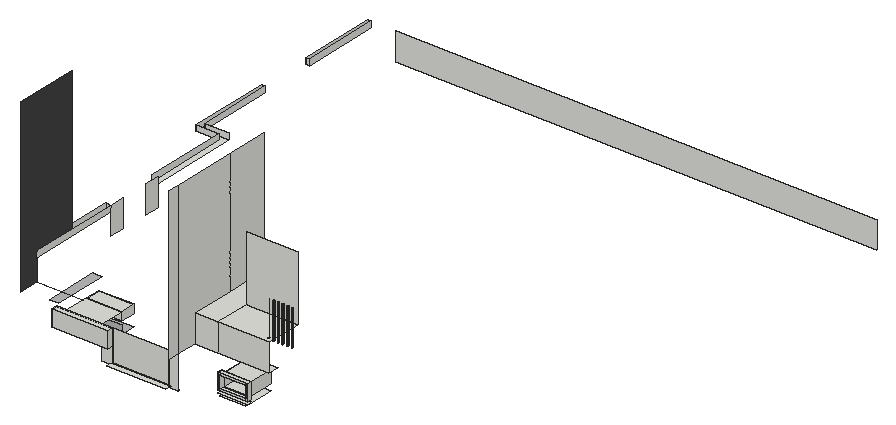
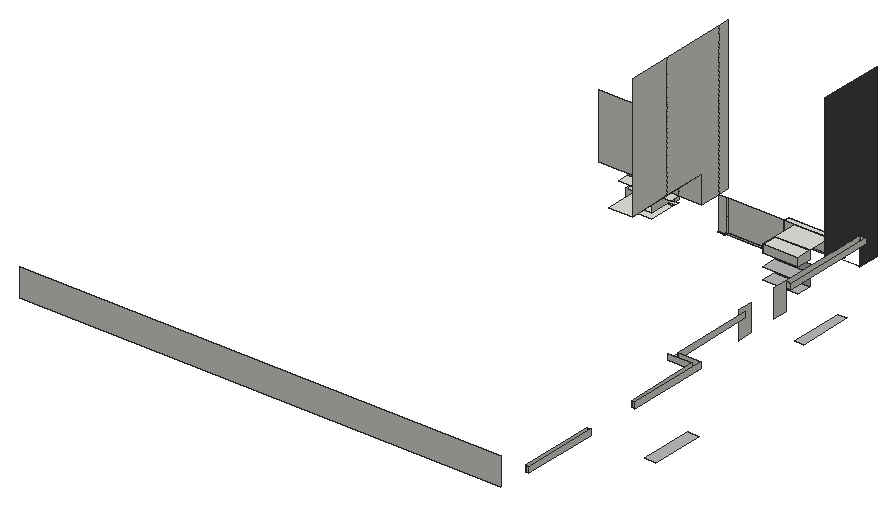
# SketchUp Ruby script. Lengths in inches.
U = 1.inch
M = Sketchup.active_model
def pt(a) = Geom::Point3d.new(a.map { |v| v * U })
def face(e, loops, mat)
  f = e.add_face(loops[0].map { |a| pt(a) })
  loops[1..].each { |l| e.add_face(l.map { |a| pt(a) }).erase! }
  f.material = f.back_material = mat if mat
  f
end
# faces: each face lists its corners as indices into pts; further lists are holes
def faces(e, pts, list, mat = nil) = list.each { |f| face(e, (f[0].is_a?(Array) ? f : [f]).map { |l| l.map { |i| pts[i] } }, mat) }
# xy, xz, yz: faces in a plane at the given z, y or x. An outline is a flat list of corners, or four numbers for a rectangle; further outlines are holes
def ring(l) = l.size == 4 ? [[l[0], l[1]], [l[2], l[1]], [l[2], l[3]], [l[0], l[3]]] : l.each_slice(2).to_a
def flat(e, list, mat, &to3) = list.each { |f| face(e, (f[0].is_a?(Array) ? f : [f]).map { |l| ring(l).map { |u, v| to3.(u, v) } }, mat) }
def xy(e, z, list, mat = nil) = flat(e, list, mat) { |x, y| [x, y, z] }
def xz(e, y, list, mat = nil) = flat(e, list, mat) { |x, z| [x, y, z] }
def yz(e, x, list, mat = nil) = flat(e, list, mat) { |y, z| [x, y, z] }
def lines(e, pts, list) = list.each { |a, b| e.add_line(pt(pts[a]), pt(pts[b])) }
# prism: a flat outline (further loops are holes) pulled along v
def prism(e, loops, v, mat = nil)
  f = face(e, loops, mat); d = Geom::Vector3d.new(v.map { |x| x * U })
  f.pushpull(f.normal.samedirection?(d) ? d.length : -d.length)
end
def box(e, o, s, mat = nil) = prism(e, [[o, [o[0] + s[0], o[1], o[2]], [o[0] + s[0], o[1] + s[1], o[2]], [o[0], o[1] + s[1], o[2]]]], [0, 0, s[2]], mat)
def at(x, y, z, deg = 0) = Geom::Transformation.translation(pt([x, y, z])) * Geom::Transformation.rotation(ORIGIN, Z_AXIS, deg.degrees)
def axes(o, x, y, z) = Geom::Transformation.new([*x, 0, *y, 0, *z, 0, *pt(o).to_a, 1])
def part(name) = M.definitions.add(name)
# library, detail: a bought-in or finely detailed component or shape, given as its bounding box
def library(name, o, s) = part(name).tap { |d| box(d.entities, o, s) }
def detail(e, o, s) = box(e.add_group.entities, o, s)
def put(e, d, t, mat = nil) = e.add_instance(d, t).tap { |i| i.material = mat if mat }
def group(e, t, mat = nil) = e.add_group.tap { |g| g.transformation = t; g.material = mat if mat }.entities
root = M.entities
M.materials.add("Generic\#2").color = [186, 186, 186]
M.materials.add("[Granite Dark Gray]").color = [68, 67, 67]
c1 = part("Group\#1")
xy(c1.entities,0,[[0,0,46.77,20.375]])
xz(c1.entities,0,[[0,0,46.77,11.0625]])
xy(root,943.1875,[[157.47,97.25,170.35,98],[249.19,97.25,259.3125,98]])
xy(root,943.6875,[[157.47,97.25,170.35,98],[249.19,97.25,259.3125,98]])
xy(root,945.84,[[170.35,89.25,249.19,97.25],[171.66,97.25,172.16,98],[247.01,97.25,247.51,98]])
xy(root,946,[[0,454.08,15.3125,525.8]],"Generic\#2")
xy(root,946.25,[[36.4375,161.95,48.5,234.18]],"Generic\#2")
xy(root,957.08,[[314.83,97.5,349.58,103.5],[314.83,103.5,349.58,138.74]])
xy(root,959.57,[[312.34,97.5,352.07,103.5]])
xy(root,962.59,[[312.34,97.5,352.07,103.5]])
xy(root,965.08,[[314.83,97.5,349.58,103.5],[314.83,103.5,349.58,138.74]])
xy(root,966.17,[[96.98,89.5625,171.66,97.25]])
xy(root,981.95,[[314.83,97.5,349.58,103.5],[314.83,103.5,349.58,138.74]])
xy(root,984.44,[[312.34,97.5,352.07,103.5]])
xy(root,987.75,[[96.98,89.5625,171.66,97.25],[110.7,97.25,157.47,130.3125],[171.66,97.25,172.16,98],[247.01,97.25,247.51,98],[290.4375,124.5,359.25,138.74],
  [110.7,130.3125,157.47,150.6875]])
xy(root,1016.8125,[[41,124.5,48.5,249],[41,326.1875,41,438.6875,10.5,438.6875,10.5,547.73,15.3125,547.73,15.3125,446.1875,48.5,446.1875,48.5,326.1875],[10.5,621.86,15.3125,724.5]])
xy(root,1024.6875,[[259.3125,124.5,290.4375,241.25],[[290.4375,124.5,359.25,172.5],[353.98,129.75,353.77,129.78,353.57,129.86,353.41,129.99,353.28,130.16,353.2,130.36,353.17,130.57,353.2,130.78,353.28,130.97,353.41,131.14,353.57,131.27,353.77,131.35,353.98,131.38,354.19,131.35,354.39,131.27,354.56,131.14,354.68,130.97,354.77,130.78,354.79,130.57,354.77,130.36,354.68,130.16,354.56,129.99,354.39,129.86,354.19,129.78]],[353.98,129.75,354.19,129.78,354.39,129.86,354.56,129.99,354.68,130.16,354.77,130.36,354.79,130.57,354.77,130.78,354.68,130.97,354.56,131.14,354.39,131.27,354.19,131.35,353.98,131.38,353.77,131.35,353.57,131.27,353.41,131.14,353.28,130.97,353.2,130.78,353.17,130.57,353.2,130.36,353.28,130.16,353.41,129.99,353.57,129.86,353.77,129.78],[360.79,129.75,360.58,129.78,360.39,129.86,360.22,129.99,360.09,130.16,360.01,130.36,359.98,130.57,360.01,130.78,360.09,130.97,360.22,131.14,360.39,131.27,360.58,131.35,360.79,131.38,361,131.35,361.2,131.27,361.37,131.14,361.5,130.97,361.58,130.78,361.61,130.57,361.58,130.36,361.5,130.16,361.37,129.99,361.2,129.86,361,129.78],[366.79,129.75,366.58,129.78,366.39,129.86,366.22,129.99,366.09,130.16,366.01,130.36,365.98,130.57,366.01,130.78,366.09,130.97,366.22,131.14,366.39,131.27,366.58,131.35,366.79,131.38,367,131.35,367.2,131.27,367.37,131.14,367.5,130.97,367.58,130.78,367.61,130.57,367.58,130.36,367.5,130.16,367.37,129.99,367.2,129.86,367,129.78],
  [372.73,129.75,372.52,129.78,372.32,129.86,372.16,129.99,372.03,130.16,371.95,130.36,371.92,130.57,371.95,130.78,372.03,130.97,372.16,131.14,372.32,131.27,372.52,131.35,372.73,131.38,372.94,131.35,373.14,131.27,373.31,131.14,373.43,130.97,373.52,130.78,373.54,130.57,373.52,130.36,373.43,130.16,373.31,129.99,373.14,129.86,372.94,129.78],[378.98,129.75,378.77,129.78,378.57,129.86,378.41,129.99,378.28,130.16,378.2,130.36,378.17,130.57,378.2,130.78,378.28,130.97,378.41,131.14,378.57,131.27,378.77,131.35,378.98,131.38,379.19,131.35,379.39,131.27,379.56,131.14,379.68,130.97,379.77,130.78,379.79,130.57,379.77,130.36,379.68,130.16,379.56,129.99,379.39,129.86,379.19,129.78],[385.23,129.75,385.02,129.78,384.82,129.86,384.66,129.99,384.53,130.16,384.45,130.36,384.42,130.57,384.45,130.78,384.53,130.97,384.66,131.14,384.82,131.27,385.02,131.35,385.23,131.38,385.44,131.35,385.64,131.27,385.81,131.14,385.93,130.97,386.02,130.78,386.04,130.57,386.02,130.36,385.93,130.16,385.81,129.99,385.64,129.86,385.44,129.78]])
xz(root,89.5625,[[96.98,966.17,171.66,987.75]])
xz(root,97.25,[[157.47,943.6875,170.35,943.6875,170.35,945.84,171.66,945.84,171.66,966.17,157.47,966.17],[170.35,943.6875,171.66,945.84],[171.66,943.6875,247.01,945.84],[247.01,943.6875,249.19,945.84],[249.19,943.6875,259.3125,943.6875,259.3125,987.75,247.51,987.75,247.51,945.84,249.19,945.84],
  [172.16,945.84,247.01,987.75],[96.98,966.17,110.7,987.75],[110.7,966.17,157.47,987.75],[157.47,966.17,171.66,987.75]])
xz(root,97.5,[[[312.34,962.59,352.07,984.44],[314.83,965.08,349.58,981.95]]])
xz(root,98,[[157.47,943.1875,170.35,943.6875],[249.19,943.1875,259.3125,943.6875],[171.66,945.84,172.16,987.75],[247.01,945.84,247.51,987.75]])
xz(root,103.5,[[[312.34,962.59,352.07,984.44],[314.83,965.08,349.58,981.95]]])
xz(root,124.5,[[259.3125,987.75,290.4375,1024.6875],[290.4375,987.75,359.25,1024.6875],[41,1016.8125,48.5,1024.6875]])
xz(root,150.6875,[[110.7,976.6875,157.47,987.75]])
xz(root,172.5,[[290.4375,1024.6875,359.25,1111.375]])
xz(root,249,[[41,1016.8125,48.5,1024.6875]])
xz(root,438.6875,[[10.5,1016.8125,41,1024.6875]])
xz(root,446.1875,[[15.3125,1016.8125,48.5,1024.6875]])
xz(root,547.73,[[10.5,1016.8125,15.3125,1024.6875]])
xz(root,621.86,[[10.5,1016.8125,15.3125,1024.6875]])
xz(root,724.5,[[48.5,987.75,690.4375,1024.6875],[10.5,1016.8125,15.3125,1024.6875]])
yz(root,10.5,[[438.6875,1016.8125,547.73,1024.6875],[621.86,1016.8125,724.5,1024.6875]])
yz(root,15.3125,[[446.1875,1016.8125,547.73,1024.6875],[621.86,1016.8125,724.5,1024.6875]])
yz(root,41,[[124.5,1016.8125,249,1024.6875],[326.1875,1016.8125,438.6875,1024.6875]])
yz(root,48.5,[[249,987.75,268.32,1024.6875],[306.87,987.75,326.1875,1024.6875],[124.5,1016.8125,249,1024.6875]])
yz(root,48.5,[[97.25,987.75,97.25,1214.9375,183.25,1214.9375,183.25,1024.6875,124.5,1024.6875,124.5,987.75]],"[Granite Dark Gray]")
yz(root,96.98,[[89.5625,966.17,97.25,987.75]])
yz(root,110.7,[[130.3125,976.6875,150.6875,987.75]])
yz(root,157.47,[[130.3125,976.6875,150.6875,987.75]])
yz(root,170.35,[[97.25,943.1875,98,943.6875]])
yz(root,171.66,[[97.25,945.84,98,966.17],[89.5625,966.17,97.25,987.75],[97.25,966.17,98,987.75]])
yz(root,172.16,[[97.25,945.84,98,966.17],[97.25,966.17,98,987.75]])
yz(root,247.01,[[97.25,945.84,98,966.17],[97.25,966.17,98,987.75]])
yz(root,247.51,[[97.25,945.84,98,966.17],[97.25,966.17,98,987.75]])
yz(root,249.19,[[97.25,943.1875,98,943.6875]])
yz(root,259.3125,[[81.125,987.75,97.25,1189.3125],[97.25,987.75,97.25,1189.3125,183.25,1189.3125,183.25,1024.6875,124.5,1024.6875,124.5,987.75],[183.25,1024.6875,241.25,1189.3125]])
yz(root,312.34,[[97.5,962.59,103.5,984.44]])
yz(root,314.83,[[97.5,965.08,103.5,981.95],[103.5,965.08,138.74,981.95]])
yz(root,349.58,[[97.5,965.08,103.5,981.95],[103.5,965.08,138.74,981.95]])
yz(root,352.07,[[97.5,962.59,103.5,984.44]])
p = [[360.39,129.86,1024.6875],[360.58,129.78,1024.6875],[360.58,129.78,1072.38],[360.39,129.86,1072.38],[360.79,129.75,1024.6875],[360.79,129.75,1072.38],
  [361,129.78,1024.6875],[361,129.78,1072.38],[361.2,129.86,1024.6875],[361.2,129.86,1072.38],[366.39,129.86,1024.6875],[366.58,129.78,1024.6875],
  [366.58,129.78,1072.38],[366.39,129.86,1072.38],[366.79,129.75,1024.6875],[366.79,129.75,1072.38],[367,129.78,1024.6875],[367,129.78,1072.38],
  [367.2,129.86,1024.6875],[367.2,129.86,1072.38],[372.32,129.86,1024.6875],[372.52,129.78,1024.6875],[372.52,129.78,1072.38],[372.32,129.86,1072.38],
  [372.73,129.75,1024.6875],[372.73,129.75,1072.38],[372.94,129.78,1024.6875],[372.94,129.78,1072.38],[373.14,129.86,1024.6875],[373.14,129.86,1072.38],
  [378.57,129.86,1024.6875],[378.77,129.78,1024.6875],[378.77,129.78,1072.38],[378.57,129.86,1072.38],[378.98,129.75,1024.6875],[378.98,129.75,1072.38],
  [379.19,129.78,1024.6875],[379.19,129.78,1072.38],[379.39,129.86,1024.6875],[379.39,129.86,1072.38],[384.82,129.86,1024.6875],[385.02,129.78,1024.6875],
  [385.02,129.78,1072.38],[384.82,129.86,1072.38],[385.23,129.75,1024.6875],[385.23,129.75,1072.38],[385.44,129.78,1024.6875],[385.44,129.78,1072.38],
  [385.64,129.86,1024.6875],[385.64,129.86,1072.38],[360.22,129.99,1024.6875],[360.22,129.99,1072.38],[361.37,129.99,1024.6875],[361.37,129.99,1072.38],
  [366.22,129.99,1024.6875],[366.22,129.99,1072.38],[367.37,129.99,1024.6875],[367.37,129.99,1072.38],[372.16,129.99,1024.6875],[372.16,129.99,1072.38],
  [373.31,129.99,1024.6875],[373.31,129.99,1072.38],[378.41,129.99,1024.6875],[378.41,129.99,1072.38],[379.56,129.99,1024.6875],[379.56,129.99,1072.38],
  [384.66,129.99,1024.6875],[384.66,129.99,1072.38],[385.81,129.99,1024.6875],[385.81,129.99,1072.38],[360.09,130.16,1024.6875],[360.09,130.16,1072.38],
  [361.5,130.16,1024.6875],[361.5,130.16,1072.38],[366.09,130.16,1024.6875],[366.09,130.16,1072.38],[367.5,130.16,1024.6875],[367.5,130.16,1072.38],
  [372.03,130.16,1024.6875],[372.03,130.16,1072.38],[373.43,130.16,1024.6875],[373.43,130.16,1072.38],[378.28,130.16,1024.6875],[378.28,130.16,1072.38],
  [379.68,130.16,1024.6875],[379.68,130.16,1072.38],[384.53,130.16,1024.6875],[384.53,130.16,1072.38],[385.93,130.16,1024.6875],[385.93,130.16,1072.38],
  [360.01,130.36,1024.6875],[360.01,130.36,1072.38],[361.58,130.36,1024.6875],[361.58,130.36,1072.38],[366.01,130.36,1024.6875],[366.01,130.36,1072.38],
  [367.58,130.36,1024.6875],[367.58,130.36,1072.38],[371.95,130.36,1024.6875],[371.95,130.36,1072.38],[373.52,130.36,1024.6875],[373.52,130.36,1072.38],
  [378.2,130.36,1024.6875],[378.2,130.36,1072.38],[379.77,130.36,1024.6875],[379.77,130.36,1072.38],[384.45,130.36,1024.6875],[384.45,130.36,1072.38],
  [386.02,130.36,1024.6875],[386.02,130.36,1072.38],[359.98,130.57,1024.6875],[359.98,130.57,1072.38],[361.61,130.57,1024.6875],[361.61,130.57,1072.38],
  [365.98,130.57,1024.6875],[365.98,130.57,1072.38],[367.61,130.57,1024.6875],[367.61,130.57,1072.38],[371.92,130.57,1024.6875],[371.92,130.57,1072.38],
  [373.54,130.57,1024.6875],[373.54,130.57,1072.38],[378.17,130.57,1024.6875],[378.17,130.57,1072.38],[379.79,130.57,1024.6875],[379.79,130.57,1072.38],
  [384.42,130.57,1024.6875],[384.42,130.57,1072.38],[386.04,130.57,1024.6875],[386.04,130.57,1072.38],[360.01,130.78,1024.6875],[360.01,130.78,1072.38],
  [361.58,130.78,1024.6875],[361.58,130.78,1072.38],[366.01,130.78,1024.6875],[366.01,130.78,1072.38],[367.58,130.78,1024.6875],[367.58,130.78,1072.38],
  [371.95,130.78,1024.6875],[371.95,130.78,1072.38],[373.52,130.78,1024.6875],[373.52,130.78,1072.38],[378.2,130.78,1024.6875],[378.2,130.78,1072.38],
  [379.77,130.78,1024.6875],[379.77,130.78,1072.38],[384.45,130.78,1024.6875],[384.45,130.78,1072.38],[360.09,130.97,1024.6875],[360.09,130.97,1072.38],
  [361.5,130.97,1024.6875],[361.5,130.97,1072.38],[366.09,130.97,1024.6875],[366.09,130.97,1072.38],[367.5,130.97,1024.6875],[367.5,130.97,1072.38],
  [372.03,130.97,1024.6875],[372.03,130.97,1072.38],[373.43,130.97,1024.6875],[373.43,130.97,1072.38],[378.28,130.97,1024.6875],[378.28,130.97,1072.38],
  [379.68,130.97,1024.6875],[379.68,130.97,1072.38],[384.53,130.97,1024.6875],[384.53,130.97,1072.38],[386.02,130.78,1024.6875],[385.93,130.97,1024.6875],
  [385.93,130.97,1072.38],[386.02,130.78,1072.38],[360.22,131.14,1024.6875],[360.22,131.14,1072.38],[361.37,131.14,1024.6875],[361.37,131.14,1072.38],
  [366.22,131.14,1024.6875],[366.22,131.14,1072.38],[367.37,131.14,1024.6875],[367.37,131.14,1072.38],[372.16,131.14,1024.6875],[372.16,131.14,1072.38],
  [373.31,131.14,1024.6875],[373.31,131.14,1072.38],[378.41,131.14,1024.6875],[378.41,131.14,1072.38],[379.56,131.14,1024.6875],[379.56,131.14,1072.38],
  [384.66,131.14,1024.6875],[384.66,131.14,1072.38],[385.81,131.14,1024.6875],[385.81,131.14,1072.38],[360.39,131.27,1024.6875],[360.39,131.27,1072.38],
  [361.2,131.27,1024.6875],[361.2,131.27,1072.38],[366.39,131.27,1024.6875],[366.39,131.27,1072.38],[367.2,131.27,1024.6875],[367.2,131.27,1072.38],
  [372.32,131.27,1024.6875],[372.32,131.27,1072.38],[373.14,131.27,1024.6875],[373.14,131.27,1072.38],[378.57,131.27,1024.6875],[378.57,131.27,1072.38],
  [379.39,131.27,1024.6875],[379.39,131.27,1072.38],[384.82,131.27,1024.6875],[384.82,131.27,1072.38],[385.64,131.27,1024.6875],[385.64,131.27,1072.38],
  [360.58,131.35,1024.6875],[360.58,131.35,1072.38],[361,131.35,1024.6875],[361,131.35,1072.38],[366.58,131.35,1024.6875],[366.58,131.35,1072.38],
  [367,131.35,1024.6875],[367,131.35,1072.38],[372.52,131.35,1024.6875],[372.52,131.35,1072.38],[372.94,131.35,1024.6875],[372.94,131.35,1072.38],
  [378.77,131.35,1024.6875],[378.77,131.35,1072.38],[379.19,131.35,1024.6875],[379.19,131.35,1072.38],[385.02,131.35,1024.6875],[385.02,131.35,1072.38],
  [385.44,131.35,1024.6875],[385.44,131.35,1072.38],[360.79,131.38,1024.6875],[360.79,131.38,1072.38],[366.79,131.38,1024.6875],[366.79,131.38,1072.38],
  [372.73,131.38,1024.6875],[372.73,131.38,1072.38],[378.98,131.38,1024.6875],[378.98,131.38,1072.38],[385.23,131.38,1024.6875],[385.23,131.38,1072.38],
  [48.5,124.5,987.75],[110.7,124.5,987.75],[385.11,130.57,1072.38],[385.11,130.57,1024.6875],[378.98,130.57,1072.38],[378.98,130.57,1024.6875],
  [372.86,130.57,1072.38],[372.86,130.57,1024.6875],[366.73,130.57,1072.38],[366.73,130.57,1024.6875],[360.61,130.57,1072.38],[360.61,130.57,1024.6875],
  [354.48,130.57,1072.38],[354.48,130.57,1024.6875]]
faces(root,p,[[0,1,2,3],[1,4,5,2],[4,6,7,5],[6,8,9,7],[10,11,12,13],[11,14,15,12],[14,16,17,15],[16,18,19,17],
  [20,21,22,23],[21,24,25,22],[24,26,27,25],[26,28,29,27],[30,31,32,33],[31,34,35,32],[34,36,37,35],[36,38,39,37],
  [40,41,42,43],[41,44,45,42],[44,46,47,45],[46,48,49,47],[50,0,3,51],[8,52,53,9],[54,10,13,55],[18,56,57,19],
  [58,20,23,59],[28,60,61,29],[62,30,33,63],[38,64,65,39],[66,40,43,67],[48,68,69,49],[70,50,51,71],[52,72,73,53],
  [74,54,55,75],[56,76,77,57],[78,58,59,79],[60,80,81,61],[82,62,63,83],[64,84,85,65],[86,66,67,87],[68,88,89,69],
  [90,70,71,91],[72,92,93,73],[94,74,75,95],[76,96,97,77],[98,78,79,99],[80,100,101,81],[102,82,83,103],[84,104,105,85],
  [106,86,87,107],[88,108,109,89],[110,90,91,111],[92,112,113,93],[114,94,95,115],[96,116,117,97],[118,98,99,119],[100,120,121,101],
  [122,102,103,123],[104,124,125,105],[126,106,107,127],[108,128,129,109],[130,110,111,131],[112,132,133,113],[134,114,115,135],[116,136,137,117],
  [138,118,119,139],[120,140,141,121],[142,122,123,143],[124,144,145,125],[146,126,127,147],[148,130,131,149],[132,150,151,133],[152,134,135,153],
  [136,154,155,137],[156,138,139,157],[140,158,159,141],[160,142,143,161],[144,162,163,145],[164,146,147,165],[166,167,168,169],[170,148,149,171],
  [150,172,173,151],[174,152,153,175],[154,176,177,155],[178,156,157,179],[158,180,181,159],[182,160,161,183],[162,184,185,163],[186,164,165,187],
  [167,188,189,168],[190,170,171,191],[172,192,193,173],[194,174,175,195],[176,196,197,177],[198,178,179,199],[180,200,201,181],[202,182,183,203],
  [184,204,205,185],[206,186,187,207],[188,208,209,189],[210,190,191,211],[192,212,213,193],[214,194,195,215],[196,216,217,197],[218,198,199,219],
  [200,220,221,201],[222,202,203,223],[204,224,225,205],[226,206,207,227],[208,228,229,209],[230,210,211,231],[212,230,231,213],[232,214,215,233],
  [216,232,233,217],[234,218,219,235],[220,234,235,221],[236,222,223,237],[224,236,237,225],[238,226,227,239],[228,238,239,229]],"Generic\#2")
lines(root,p,[[240,241],[242,243],[244,245],[246,247],[248,249],[250,251],[252,253]])
put(root,c1,at(110.7,130.3125,944.3125),"Generic\#2")
put(root,c1,at(110.7,130.3125,960.5),"Generic\#2")
put(root,c1,at(110.7,130.3125,976.6875))
